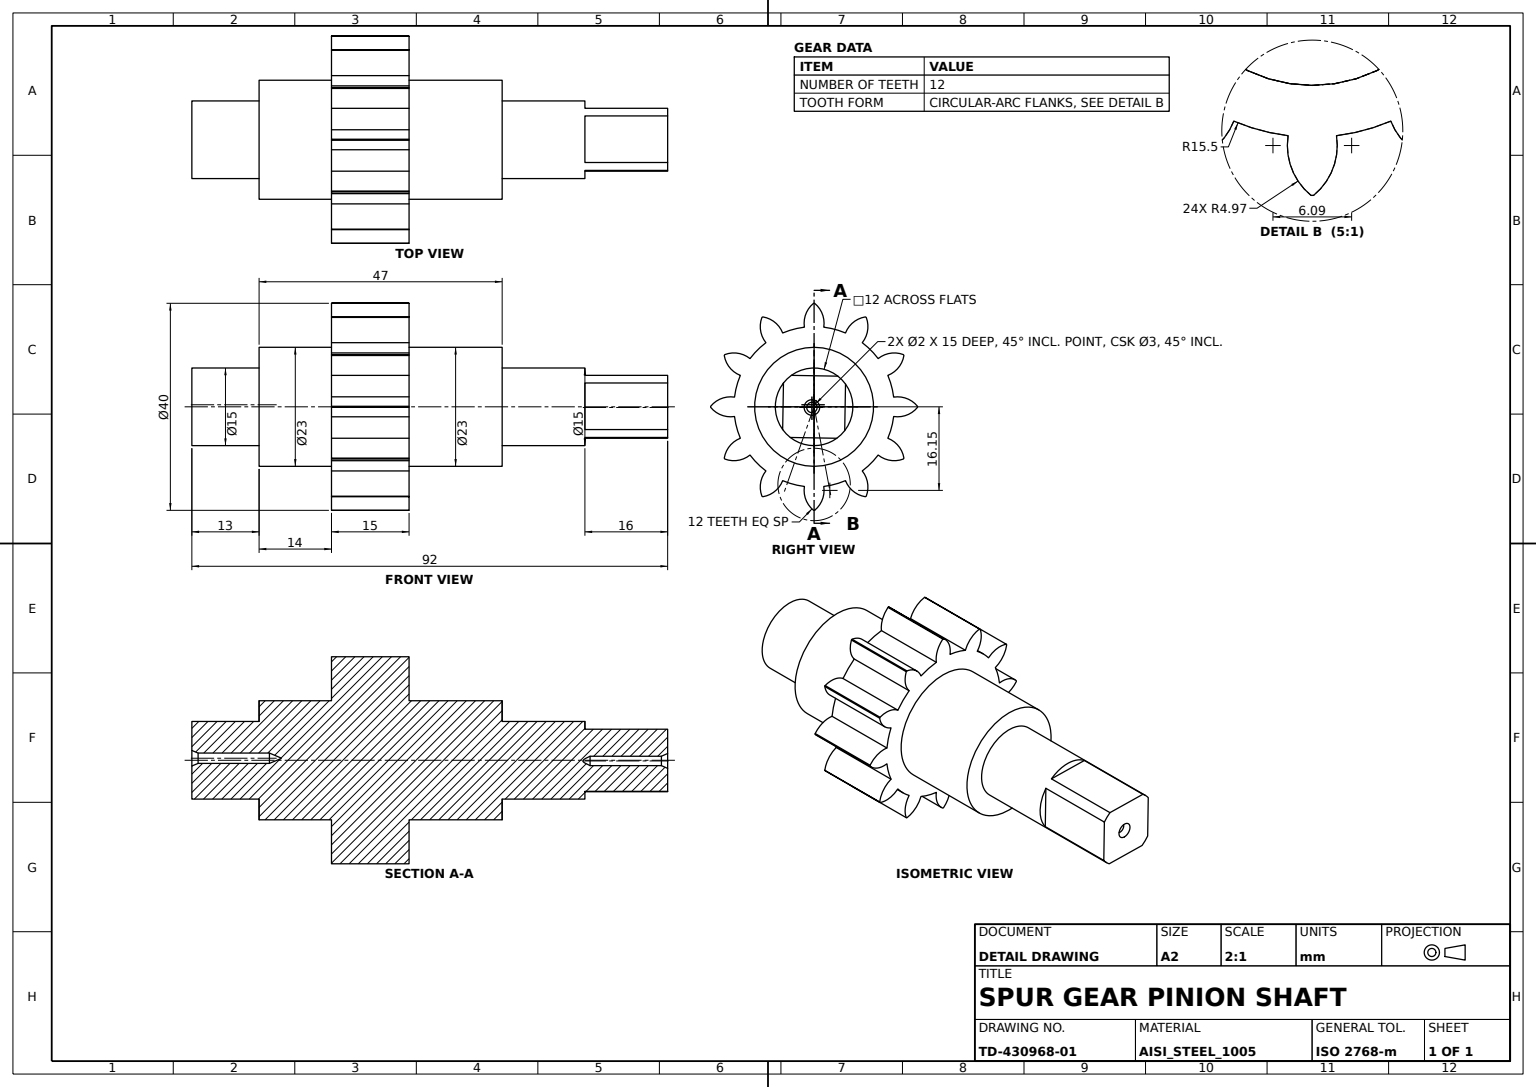
solid
v1 (0,-21.5,-11.5)
e1 v1 v1 CIRCLE(AX(P(0,-21.5,0),D(0,-1,0),D(0,0,-1)),11.5)
v2 (0,-7.5,-11.5)
e2 v2 v2 CIRCLE(AX(P(0,-7.5,0),D(0,-1,0),D(0,0,-1)),11.5)
face CYL(AX(P(0,0,0),D(0,-1,0),D(0,0,-1)),11.5) [-e1] [e2]
v3 (-1.87227,7.5,-15.386507)
v4 (-0.10064,7.5,-19.999747)
e3 v3 v4 CIRCLE(AX(P(3.042634,7.5,-16.14583),D(0,-1,0),D(1,0,0)),4.973213)
v5 (-0.10064,-7.5,-19.999747)
e4 v5 v4 LINE
v6 (-1.87227,-7.5,-15.386507)
e5 v6 v5 CIRCLE(AX(P(3.042634,-7.5,-16.14583),D(0,1,0),D(0,0,1)),4.973213) rev
e6 v3 v6 LINE
face CYL(AX(P(3.042634,-42.5,-16.14583),D(0,1,0),D(0,0,1)),4.973213) [e3 -e4 -e5 -e6]
v7 (14.261241,7.5,-6.071821)
v8 (15.386507,7.5,-1.87227)
e7 v7 v8 CIRCLE(AX(P(0,7.5,0),D(0,-1,0),D(1,0,0)),15.5)
v9 (15.386507,-7.5,-1.87227)
e8 v8 v9 LINE
v10 (14.261241,-7.5,-6.071821)
e9 v10 v9 CIRCLE(AX(P(0,-7.5,0),D(0,1,0),D(0,0,1)),15.5) rev
e10 v7 v10 LINE
face CYL(AX(P(0,-42.5,0),D(0,1,0),D(0,0,1)),15.5) [e7 e8 -e9 -e10]
v11 (0,-34.5,-7.5)
e11 v11 v11 CIRCLE(AX(P(0,-34.5,0),D(0,-1,0),D(0,0,-1)),7.5)
v12 (0,-21.5,-7.5)
e12 v12 v12 CIRCLE(AX(P(0,-21.5,0),D(0,-1,0),D(0,0,-1)),7.5)
face CYL(AX(P(0,0,0),D(0,-1,0),D(0,0,-1)),7.5) [-e11] [e12]
v13 (12.388971,7.5,9.314687)
v14 (9.314687,7.5,12.388971)
e13 v13 v14 CIRCLE(AX(P(0,7.5,0),D(0,-1,0),D(1,0,0)),15.5)
v15 (9.314687,-7.5,12.388971)
e14 v14 v15 LINE
v16 (12.388971,-7.5,9.314687)
e15 v16 v15 CIRCLE(AX(P(0,-7.5,0),D(0,1,0),D(0,0,1)),15.5) rev
e16 v13 v16 LINE
face CYL(AX(P(0,-42.5,0),D(0,1,0),D(0,0,1)),15.5) [e13 e14 -e15 -e16]
v17 (5.92055,41.5,4.604029)
v18 (5.92055,57.5,4.604029)
e17 v17 v18 LINE
v19 (6.077622,41.5,-4.3946)
e18 v17 v19 LINE
v20 (6.077622,57.5,-4.3946)
e19 v20 v19 LINE
e20 v20 v18 LINE
face PLANE(AX(P(6.077622,41.5,-4.3946),D(-0.999847695,0,-0.017452406),D(-0.017452406,0,0.999847695))) rev [-e17 e18 -e19 e20]
v21 (-9.912717,-7.5,17.370609)
v22 (-9.912717,7.5,17.370609)
e21 v21 v22 LINE
v23 (-6.071821,-7.5,14.261241)
e22 v23 v21 CIRCLE(AX(P(-10.707913,-7.5,12.461382),D(0,1,0),D(0,0,1)),4.973213) rev
v24 (-6.071821,7.5,14.261241)
e23 v24 v23 LINE
e24 v24 v22 CIRCLE(AX(P(-10.707913,7.5,12.461382),D(0,-1,0),D(-0.866025404,0,-0.5)),4.973213)
face CYL(AX(P(-10.707913,-42.5,12.461382),D(0,1,0),D(0,0,1)),4.973213) [-e21 -e22 -e23 e24]
v25 (-6.071821,7.5,-14.261241)
e25 v25 v3 CIRCLE(AX(P(0,7.5,0),D(0,-1,0),D(1,0,0)),15.5)
v26 (-6.071821,-7.5,-14.261241)
e26 v26 v6 CIRCLE(AX(P(0,-7.5,0),D(0,1,0),D(0,0,1)),15.5) rev
e27 v25 v26 LINE
face CYL(AX(P(0,-42.5,0),D(0,1,0),D(0,0,1)),15.5) [e25 e6 -e26 -e27]
v27 (9.314687,7.5,-12.388971)
v28 (9.314687,-7.5,-12.388971)
e28 v27 v28 LINE
v29 (10.08703,-7.5,-17.269969)
e29 v29 v28 CIRCLE(AX(P(5.437917,-7.5,-15.504016),D(0,1,0),D(0,0,1)),4.973213) rev
v30 (10.08703,7.5,-17.269969)
e30 v29 v30 LINE
e31 v30 v27 CIRCLE(AX(P(5.437917,7.5,-15.504016),D(0,-1,0),D(-0.866025404,0,-0.5)),4.973213)
face CYL(AX(P(5.437917,-42.5,-15.504016),D(0,1,0),D(0,0,1)),4.973213) [e28 -e29 e30 e31]
v31 (9.912717,7.5,17.370609)
v32 (6.071821,7.5,14.261241)
e32 v31 v32 CIRCLE(AX(P(10.707913,7.5,12.461382),D(0,-1,0),D(0.866025404,0,-0.5)),4.973213)
v33 (6.071821,-7.5,14.261241)
e33 v32 v33 LINE
v34 (9.912717,-7.5,17.370609)
e34 v34 v33 CIRCLE(AX(P(10.707913,-7.5,12.461382),D(0,1,0),D(0,0,1)),4.973213) rev
e35 v34 v31 LINE
face CYL(AX(P(10.707913,-42.5,12.461382),D(0,1,0),D(0,0,1)),4.973213) [e32 e33 -e34 e35]
v35 (0.421315,56.292893,-1.128229)
e36 v35 v35 CIRCLE(AX(P(0.421315,56.292893,-0.128229),D(0,-1,0),D(0,0,-1)),1) rev
v36 (0.421315,57.5,-1.628229)
e37 v36 v36 CIRCLE(AX(P(0.421315,57.5,-0.128229),D(0,-1,0),D(0,0,-1)),1.5)
face CONE(AX(P(0.421315,57.5,-0.128229),D(0,1,0),D(0,0,1)),1.5,0.392699082) rev [-e36] [-e37]
v37 (-14.261241,7.5,6.071821)
v38 (-14.261241,-7.5,6.071821)
e38 v37 v38 LINE
v39 (-17.370609,-7.5,9.912717)
e39 v39 v38 CIRCLE(AX(P(-12.461382,-7.5,10.707913),D(0,1,0),D(0,0,1)),4.973213) rev
v40 (-17.370609,7.5,9.912717)
e40 v39 v40 LINE
e41 v40 v37 CIRCLE(AX(P(-12.461382,7.5,10.707913),D(0,-1,0),D(0.5,0,0.866025404)),4.973213)
face CYL(AX(P(-12.461382,-42.5,10.707913),D(0,1,0),D(0,0,1)),4.973213) [e38 -e39 e40 e41]
v41 (1.87227,-7.5,15.386507)
v42 (0.10064,-7.5,19.999747)
e42 v41 v42 CIRCLE(AX(P(-3.042634,-7.5,16.14583),D(0,1,0),D(0,0,1)),4.973213) rev
v43 (1.87227,7.5,15.386507)
e43 v43 v41 LINE
v44 (0.10064,7.5,19.999747)
e44 v43 v44 CIRCLE(AX(P(-3.042634,7.5,16.14583),D(0,-1,0),D(-1,0,0)),4.973213)
e45 v42 v44 LINE
face CYL(AX(P(-3.042634,-42.5,16.14583),D(0,1,0),D(0,0,1)),4.973213) [-e42 -e43 e44 -e45]
v45 (0.043925,-19.5,1.395321)
e46 v45 v45 CIRCLE(AX(P(0.043925,-19.5,0.395321),D(0,1,0),D(0,0,1)),1) rev
v46 (0.043925,-33.292893,1.395321)
e47 v46 v46 CIRCLE(AX(P(0.043925,-33.292893,0.395321),D(0,1,0),D(0,0,1)),1) rev
face CYL(AX(P(0.043925,-19.5,0.395321),D(0,1,0),D(0,0,1)),1) rev [-e46] [e47]
v47 (19.999747,7.5,-0.10064)
e48 v8 v47 CIRCLE(AX(P(16.14583,7.5,3.042634),D(0,-1,0),D(0,0,1)),4.973213)
v48 (19.999747,-7.5,-0.10064)
e49 v48 v47 LINE
e50 v9 v48 CIRCLE(AX(P(16.14583,-7.5,3.042634),D(0,1,0),D(0,0,1)),4.973213) rev
face CYL(AX(P(16.14583,-42.5,3.042634),D(0,1,0),D(0,0,1)),4.973213) [-e8 e48 -e49 -e50]
v49 (-5.92055,41.5,-4.604029)
v50 (-6.077622,41.5,4.3946)
e51 v49 v50 LINE
e52 v49 v50 CIRCLE(AX(P(0,41.5,0),D(0,1,0),D(0,0,-1)),7.5)
face PLANE(AX(P(0,41.5,0),D(0,1,0),D(0,0,1))) [-e51 e52]
v51 (10.08703,-7.5,17.269969)
e53 v51 v34 CIRCLE(AX(P(0,-7.5,0),D(0,-1,0),D(0,0,-1)),20)
v52 (10.08703,7.5,17.269969)
e54 v51 v52 LINE
e55 v52 v31 CIRCLE(AX(P(0,7.5,0),D(0,-1,0),D(0,0,-1)),20)
face CYL(AX(P(0,0,0),D(0,-1,0),D(0,0,-1)),20) [-e35 -e53 e54 e55]
v53 (-4.604029,41.5,5.92055)
v54 (4.3946,41.5,6.077622)
e56 v53 v54 CIRCLE(AX(P(0,41.5,0),D(0,1,0),D(0,0,-1)),7.5)
e57 v53 v54 LINE
face PLANE(AX(P(0,41.5,0),D(0,1,0),D(0,0,1))) [e56 -e57]
v55 (-17.370609,-7.5,-9.912717)
v56 (-17.370609,7.5,-9.912717)
e58 v55 v56 LINE
v57 (-14.261241,-7.5,-6.071821)
e59 v57 v55 CIRCLE(AX(P(-12.461382,-7.5,-10.707913),D(0,1,0),D(0,0,1)),4.973213) rev
v58 (-14.261241,7.5,-6.071821)
e60 v58 v57 LINE
e61 v58 v56 CIRCLE(AX(P(-12.461382,7.5,-10.707913),D(0,-1,0),D(0.5,0,-0.866025404)),4.973213)
face CYL(AX(P(-12.461382,-42.5,-10.707913),D(0,1,0),D(0,0,1)),4.973213) [-e58 -e59 -e60 e61]
v59 (-10.08703,7.5,17.269969)
e62 v22 v59 CIRCLE(AX(P(0,7.5,0),D(0,-1,0),D(0,0,-1)),20)
v60 (-10.08703,-7.5,17.269969)
e63 v60 v59 LINE
e64 v21 v60 CIRCLE(AX(P(0,-7.5,0),D(0,-1,0),D(0,0,-1)),20)
face CYL(AX(P(0,0,0),D(0,-1,0),D(0,0,-1)),20) [e62 -e63 -e64 e21]
v61 (19.999747,-7.5,0.10064)
v62 (15.386507,-7.5,1.87227)
e65 v61 v62 CIRCLE(AX(P(16.14583,-7.5,-3.042634),D(0,1,0),D(0,0,1)),4.973213) rev
v63 (19.999747,7.5,0.10064)
e66 v61 v63 LINE
v64 (15.386507,7.5,1.87227)
e67 v63 v64 CIRCLE(AX(P(16.14583,7.5,-3.042634),D(0,-1,0),D(0,0,-1)),4.973213)
e68 v64 v62 LINE
face CYL(AX(P(16.14583,-42.5,-3.042634),D(0,1,0),D(0,0,1)),4.973213) [-e65 e66 e67 e68]
v65 (12.388971,-7.5,-9.314687)
e69 v28 v65 CIRCLE(AX(P(0,-7.5,0),D(0,1,0),D(0,0,1)),15.5) rev
v66 (17.269969,-7.5,-10.08703)
e70 v65 v66 CIRCLE(AX(P(15.504016,-7.5,-5.437917),D(0,1,0),D(0,0,1)),4.973213) rev
v67 (17.370609,-7.5,-9.912717)
e71 v66 v67 CIRCLE(AX(P(0,-7.5,0),D(0,-1,0),D(0,0,-1)),20)
e72 v67 v10 CIRCLE(AX(P(12.461382,-7.5,-10.707913),D(0,1,0),D(0,0,1)),4.973213) rev
e73 v48 v61 CIRCLE(AX(P(0,-7.5,0),D(0,-1,0),D(0,0,-1)),20)
v68 (14.261241,-7.5,6.071821)
e74 v62 v68 CIRCLE(AX(P(0,-7.5,0),D(0,1,0),D(0,0,1)),15.5) rev
v69 (17.370609,-7.5,9.912717)
e75 v68 v69 CIRCLE(AX(P(12.461382,-7.5,10.707913),D(0,1,0),D(0,0,1)),4.973213) rev
v70 (17.269969,-7.5,10.08703)
e76 v69 v70 CIRCLE(AX(P(0,-7.5,0),D(0,-1,0),D(0,0,-1)),20)
e77 v70 v16 CIRCLE(AX(P(15.504016,-7.5,5.437917),D(0,1,0),D(0,0,1)),4.973213) rev
e78 v15 v51 CIRCLE(AX(P(5.437917,-7.5,15.504016),D(0,1,0),D(0,0,1)),4.973213) rev
e79 v33 v41 CIRCLE(AX(P(0,-7.5,0),D(0,1,0),D(0,0,1)),15.5) rev
v71 (-0.10064,-7.5,19.999747)
e80 v42 v71 CIRCLE(AX(P(0,-7.5,0),D(0,-1,0),D(0,0,-1)),20)
v72 (-1.87227,-7.5,15.386507)
e81 v71 v72 CIRCLE(AX(P(3.042634,-7.5,16.14583),D(0,1,0),D(0,0,1)),4.973213) rev
e82 v72 v23 CIRCLE(AX(P(0,-7.5,0),D(0,1,0),D(0,0,1)),15.5) rev
v73 (-9.314687,-7.5,12.388971)
e83 v60 v73 CIRCLE(AX(P(-5.437917,-7.5,15.504016),D(0,1,0),D(0,0,1)),4.973213) rev
v74 (-12.388971,-7.5,9.314687)
e84 v73 v74 CIRCLE(AX(P(0,-7.5,0),D(0,1,0),D(0,0,1)),15.5) rev
v75 (-17.269969,-7.5,10.08703)
e85 v74 v75 CIRCLE(AX(P(-15.504016,-7.5,5.437917),D(0,1,0),D(0,0,1)),4.973213) rev
e86 v75 v39 CIRCLE(AX(P(0,-7.5,0),D(0,-1,0),D(0,0,-1)),20)
v76 (-15.386507,-7.5,1.87227)
e87 v38 v76 CIRCLE(AX(P(0,-7.5,0),D(0,1,0),D(0,0,1)),15.5) rev
v77 (-19.999747,-7.5,0.10064)
e88 v76 v77 CIRCLE(AX(P(-16.14583,-7.5,-3.042634),D(0,1,0),D(0,0,1)),4.973213) rev
v78 (-19.999747,-7.5,-0.10064)
e89 v77 v78 CIRCLE(AX(P(0,-7.5,0),D(0,-1,0),D(0,0,-1)),20)
v79 (-15.386507,-7.5,-1.87227)
e90 v78 v79 CIRCLE(AX(P(-16.14583,-7.5,3.042634),D(0,1,0),D(0,0,1)),4.973213) rev
e91 v79 v57 CIRCLE(AX(P(0,-7.5,0),D(0,1,0),D(0,0,1)),15.5) rev
v80 (-17.269969,-7.5,-10.08703)
e92 v55 v80 CIRCLE(AX(P(0,-7.5,0),D(0,-1,0),D(0,0,-1)),20)
v81 (-12.388971,-7.5,-9.314687)
e93 v80 v81 CIRCLE(AX(P(-15.504016,-7.5,-5.437917),D(0,1,0),D(0,0,1)),4.973213) rev
v82 (-9.314687,-7.5,-12.388971)
e94 v81 v82 CIRCLE(AX(P(0,-7.5,0),D(0,1,0),D(0,0,1)),15.5) rev
v83 (-10.08703,-7.5,-17.269969)
e95 v82 v83 CIRCLE(AX(P(-5.437917,-7.5,-15.504016),D(0,1,0),D(0,0,1)),4.973213) rev
v84 (-9.912717,-7.5,-17.370609)
e96 v83 v84 CIRCLE(AX(P(0,-7.5,0),D(0,-1,0),D(0,0,-1)),20)
e97 v84 v26 CIRCLE(AX(P(-10.707913,-7.5,-12.461382),D(0,1,0),D(0,0,1)),4.973213) rev
v85 (0.10064,-7.5,-19.999747)
e98 v5 v85 CIRCLE(AX(P(0,-7.5,0),D(0,-1,0),D(0,0,-1)),20)
v86 (1.87227,-7.5,-15.386507)
e99 v85 v86 CIRCLE(AX(P(-3.042634,-7.5,-16.14583),D(0,1,0),D(0,0,1)),4.973213) rev
v87 (6.071821,-7.5,-14.261241)
e100 v86 v87 CIRCLE(AX(P(0,-7.5,0),D(0,1,0),D(0,0,1)),15.5) rev
v88 (9.912717,-7.5,-17.370609)
e101 v87 v88 CIRCLE(AX(P(10.707913,-7.5,-12.461382),D(0,1,0),D(0,0,1)),4.973213) rev
e102 v88 v29 CIRCLE(AX(P(0,-7.5,0),D(0,-1,0),D(0,0,-1)),20)
face PLANE(AX(P(-20,-7.5,0),D(0,1,0),D(0,0,1))) rev [e69 e70 e71 e72 e9 e50 e73 e65 e74 e75 e76 e77 e15 e78 e53 e34 e79 e42 e80 e81 e82 e22 e64 e83 e84 e85 e86 e39 e87 e88 e89 e90 e91 e59 e92 e93 e94 e95 e96 e97 e26 e5 e98 e99 e100 e101 e102 e29] [-e2]
v89 (-6.077622,57.5,4.3946)
e103 v50 v89 LINE
v90 (-5.92055,57.5,-4.604029)
e104 v89 v90 LINE
e105 v90 v49 LINE
face PLANE(AX(P(-6.077622,41.5,4.3946),D(0.999847695,0,0.017452406),D(0.017452406,0,-0.999847695))) rev [e51 e103 e104 e105]
v91 (4.3946,57.5,6.077622)
e106 v54 v91 LINE
v92 (-4.604029,57.5,5.92055)
e107 v91 v92 LINE
e108 v92 v53 LINE
face PLANE(AX(P(4.3946,41.5,6.077622),D(0.017452406,0,-0.999847695),D(-0.999847695,0,-0.017452406))) rev [e57 e106 e107 e108]
v93 (17.269969,7.5,-10.08703)
e109 v66 v93 LINE
v94 (17.370609,7.5,-9.912717)
e110 v93 v94 CIRCLE(AX(P(0,7.5,0),D(0,-1,0),D(0,0,-1)),20)
e111 v67 v94 LINE
face CYL(AX(P(0,0,0),D(0,-1,0),D(0,0,-1)),20) [e109 e110 -e111 -e71]
v95 (17.269969,7.5,10.08703)
e112 v70 v95 LINE
e113 v95 v13 CIRCLE(AX(P(15.504016,7.5,5.437917),D(0,-1,0),D(0.5,0,-0.866025404)),4.973213)
face CYL(AX(P(15.504016,-42.5,5.437917),D(0,1,0),D(0,0,1)),4.973213) [e112 e113 e16 -e77]
v96 (0,25.5,-11.5)
e114 v96 v96 CIRCLE(AX(P(0,25.5,0),D(0,-1,0),D(0,0,-1)),11.5)
v97 (0,25.5,-7.5)
e115 v97 v97 CIRCLE(AX(P(0,25.5,0),D(0,-1,0),D(0,0,-1)),7.5)
face PLANE(AX(P(-7.5,25.5,0),D(0,-1,0),D(0,0,-1))) rev [-e114] [e115]
e116 v18 v91 CIRCLE(AX(P(0,57.5,0),D(0,-1,0),D(0,0,-1)),7.5)
v98 (4.604029,57.5,-5.92055)
e117 v98 v20 CIRCLE(AX(P(0,57.5,0),D(0,-1,0),D(0,0,-1)),7.5)
v99 (-4.3946,57.5,-6.077622)
e118 v99 v98 LINE
e119 v90 v99 CIRCLE(AX(P(0,57.5,0),D(0,-1,0),D(0,0,-1)),7.5)
e120 v92 v89 CIRCLE(AX(P(0,57.5,0),D(0,-1,0),D(0,0,-1)),7.5)
face PLANE(AX(P(0,57.5,0),D(0,-1,0),D(0,0,-1))) rev [-e107 -e116 -e20 -e117 -e118 -e119 -e104 -e120] [e37]
e121 v47 v63 CIRCLE(AX(P(0,7.5,0),D(0,-1,0),D(0,0,-1)),20)
face CYL(AX(P(0,0,0),D(0,-1,0),D(0,0,-1)),20) [e121 -e66 -e73 e49]
e122 v32 v43 CIRCLE(AX(P(0,7.5,0),D(0,-1,0),D(1,0,0)),15.5)
face CYL(AX(P(0,-42.5,0),D(0,1,0),D(0,0,1)),15.5) [e43 -e79 -e33 e122]
v100 (9.912717,7.5,-17.370609)
e123 v100 v30 CIRCLE(AX(P(0,7.5,0),D(0,-1,0),D(0,0,-1)),20)
e124 v88 v100 LINE
face CYL(AX(P(0,0,0),D(0,-1,0),D(0,0,-1)),20) [e123 -e30 -e102 e124]
v101 (-15.386507,7.5,1.87227)
e125 v101 v76 LINE
v102 (-19.999747,7.5,0.10064)
e126 v101 v102 CIRCLE(AX(P(-16.14583,7.5,-3.042634),D(0,-1,0),D(0,0,-1)),4.973213)
e127 v77 v102 LINE
face CYL(AX(P(-16.14583,-42.5,-3.042634),D(0,1,0),D(0,0,1)),4.973213) [-e88 -e125 e126 -e127]
v103 (1.87227,7.5,-15.386507)
e128 v103 v86 LINE
v104 (0.10064,7.5,-19.999747)
e129 v85 v104 LINE
e130 v104 v103 CIRCLE(AX(P(-3.042634,7.5,-16.14583),D(0,-1,0),D(-1,0,0)),4.973213)
face CYL(AX(P(-3.042634,-42.5,-16.14583),D(0,1,0),D(0,0,1)),4.973213) [e128 -e99 e129 e130]
v105 (-17.269969,7.5,10.08703)
e131 v75 v105 LINE
e132 v105 v40 CIRCLE(AX(P(0,7.5,0),D(0,-1,0),D(0,0,-1)),20)
face CYL(AX(P(0,0,0),D(0,-1,0),D(0,0,-1)),20) [-e86 e131 e132 -e40]
face PLANE(AX(P(-11.5,-21.5,0),D(0,1,0),D(0,0,1))) rev [e1] [-e12]
v106 (0.421315,42.5,-1.128229)
e133 v106 v106 CIRCLE(AX(P(0.421315,42.5,-0.128229),D(0,-1,0),D(0,0,-1)),1) rev
face CYL(AX(P(0.421315,42.5,-0.128229),D(0,-1,0),D(0,0,-1)),1) rev [-e133] [e36]
v107 (-4.3946,41.5,-6.077622)
e134 v99 v107 LINE
v108 (4.604029,41.5,-5.92055)
e135 v108 v107 CIRCLE(AX(P(0,41.5,0),D(0,1,0),D(0,0,-1)),7.5)
e136 v108 v98 LINE
e137 v17 v19 CIRCLE(AX(P(0,41.5,0),D(0,1,0),D(0,0,-1)),7.5)
face CYL(AX(P(0,0,0),D(0,-1,0),D(0,0,-1)),7.5) [e116 -e106 -e56 -e108 e120 -e103 -e52 -e105 e119 e134 -e135 e136 e117 e19 -e137 e17] [-e115]
v109 (-0.10064,7.5,19.999747)
v110 (-1.87227,7.5,15.386507)
e138 v109 v110 CIRCLE(AX(P(3.042634,7.5,16.14583),D(0,-1,0),D(1,0,0)),4.973213)
e139 v110 v72 LINE
e140 v71 v109 LINE
face CYL(AX(P(3.042634,-42.5,16.14583),D(0,1,0),D(0,0,1)),4.973213) [e138 e139 -e81 e140]
v111 (14.261241,7.5,6.071821)
v112 (17.370609,7.5,9.912717)
e141 v111 v112 CIRCLE(AX(P(12.461382,7.5,10.707913),D(0,-1,0),D(-0.5,0,0.866025404)),4.973213)
e142 v69 v112 LINE
e143 v111 v68 LINE
face CYL(AX(P(12.461382,-42.5,10.707913),D(0,1,0),D(0,0,1)),4.973213) [e141 -e142 -e75 -e143]
v113 (0.043925,-34.5,1.895321)
e144 v113 v113 CIRCLE(AX(P(0.043925,-34.5,0.395321),D(0,1,0),D(0,0,1)),1.5)
face CONE(AX(P(0.043925,-34.5,0.395321),D(0,-1,0),D(0,0,-1)),1.5,0.392699082) rev [-e47] [-e144]
v114 (0.043925,-17.085786,0.395321)
face CONE(AX(P(0.043925,-19.5,0.395321),D(0,-1,0),D(0,0,-1)),1,0.392699082) rev [e46] [v114]
v115 (-19.999747,7.5,-0.10064)
e145 v78 v115 LINE
v116 (-15.386507,7.5,-1.87227)
e146 v115 v116 CIRCLE(AX(P(-16.14583,7.5,3.042634),D(0,-1,0),D(0,0,1)),4.973213)
e147 v116 v79 LINE
face CYL(AX(P(-16.14583,-42.5,3.042634),D(0,1,0),D(0,0,1)),4.973213) [e145 e146 e147 -e90]
e148 v37 v101 CIRCLE(AX(P(0,7.5,0),D(0,-1,0),D(1,0,0)),15.5)
face CYL(AX(P(0,-42.5,0),D(0,1,0),D(0,0,1)),15.5) [-e38 e148 e125 -e87]
v117 (6.071821,7.5,-14.261241)
e149 v117 v87 LINE
e150 v117 v100 CIRCLE(AX(P(10.707913,7.5,-12.461382),D(0,-1,0),D(0.866025404,0,0.5)),4.973213)
face CYL(AX(P(10.707913,-42.5,-12.461382),D(0,1,0),D(0,0,1)),4.973213) [-e124 -e101 -e149 e150]
e151 v4 v104 CIRCLE(AX(P(0,7.5,0),D(0,-1,0),D(0,0,-1)),20)
face CYL(AX(P(0,0,0),D(0,-1,0),D(0,0,-1)),20) [e4 e151 -e129 -e98]
e152 v112 v95 CIRCLE(AX(P(0,7.5,0),D(0,-1,0),D(0,0,-1)),20)
face CYL(AX(P(0,0,0),D(0,-1,0),D(0,0,-1)),20) [-e76 e142 e152 -e112]
v118 (0,7.5,-11.5)
e153 v118 v118 CIRCLE(AX(P(0,7.5,0),D(0,-1,0),D(0,0,-1)),11.5)
face CYL(AX(P(0,0,0),D(0,-1,0),D(0,0,-1)),11.5) [e114] [-e153]
e154 v102 v115 CIRCLE(AX(P(0,7.5,0),D(0,-1,0),D(0,0,-1)),20)
face CYL(AX(P(0,0,0),D(0,-1,0),D(0,0,-1)),20) [-e145 -e89 e127 e154]
v119 (-10.08703,7.5,-17.269969)
e155 v83 v119 LINE
v120 (-9.912717,7.5,-17.370609)
e156 v119 v120 CIRCLE(AX(P(0,7.5,0),D(0,-1,0),D(0,0,-1)),20)
e157 v84 v120 LINE
face CYL(AX(P(0,0,0),D(0,-1,0),D(0,0,-1)),20) [e155 e156 -e157 -e96]
v121 (12.388971,7.5,-9.314687)
e158 v121 v65 LINE
e159 v27 v121 CIRCLE(AX(P(0,7.5,0),D(0,-1,0),D(1,0,0)),15.5)
face CYL(AX(P(0,-42.5,0),D(0,1,0),D(0,0,1)),15.5) [e158 -e69 -e28 e159]
e160 v110 v24 CIRCLE(AX(P(0,7.5,0),D(0,-1,0),D(1,0,0)),15.5)
face CYL(AX(P(0,-42.5,0),D(0,1,0),D(0,0,1)),15.5) [e160 e23 -e82 -e139]
v122 (-12.388971,7.5,9.314687)
e161 v122 v105 CIRCLE(AX(P(-15.504016,7.5,5.437917),D(0,-1,0),D(-0.5,0,-0.866025404)),4.973213)
v123 (-9.314687,7.5,12.388971)
e162 v123 v122 CIRCLE(AX(P(0,7.5,0),D(0,-1,0),D(1,0,0)),15.5)
e163 v59 v123 CIRCLE(AX(P(-5.437917,7.5,15.504016),D(0,-1,0),D(0.866025404,0,0.5)),4.973213)
e164 v44 v109 CIRCLE(AX(P(0,7.5,0),D(0,-1,0),D(0,0,-1)),20)
e165 v14 v52 CIRCLE(AX(P(5.437917,7.5,15.504016),D(0,-1,0),D(-0.866025404,0,0.5)),4.973213)
e166 v64 v111 CIRCLE(AX(P(0,7.5,0),D(0,-1,0),D(1,0,0)),15.5)
e167 v94 v7 CIRCLE(AX(P(12.461382,7.5,-10.707913),D(0,-1,0),D(-0.5,0,-0.866025404)),4.973213)
e168 v121 v93 CIRCLE(AX(P(15.504016,7.5,-5.437917),D(0,-1,0),D(0.5,0,0.866025404)),4.973213)
e169 v103 v117 CIRCLE(AX(P(0,7.5,0),D(0,-1,0),D(1,0,0)),15.5)
e170 v120 v25 CIRCLE(AX(P(-10.707913,7.5,-12.461382),D(0,-1,0),D(-0.866025404,0,0.5)),4.973213)
v124 (-9.314687,7.5,-12.388971)
e171 v124 v119 CIRCLE(AX(P(-5.437917,7.5,-15.504016),D(0,-1,0),D(0.866025404,0,-0.5)),4.973213)
v125 (-12.388971,7.5,-9.314687)
e172 v125 v124 CIRCLE(AX(P(0,7.5,0),D(0,-1,0),D(1,0,0)),15.5)
v126 (-17.269969,7.5,-10.08703)
e173 v126 v125 CIRCLE(AX(P(-15.504016,7.5,-5.437917),D(0,-1,0),D(-0.5,0,0.866025404)),4.973213)
e174 v56 v126 CIRCLE(AX(P(0,7.5,0),D(0,-1,0),D(0,0,-1)),20)
e175 v116 v58 CIRCLE(AX(P(0,7.5,0),D(0,-1,0),D(1,0,0)),15.5)
face PLANE(AX(P(-11.5,7.5,0),D(0,-1,0),D(0,0,-1))) rev [e153] [-e154 -e126 -e148 -e41 -e132 -e161 -e162 -e163 -e62 -e24 -e160 -e138 -e164 -e44 -e122 -e32 -e55 -e165 -e13 -e113 -e152 -e141 -e166 -e67 -e121 -e48 -e7 -e167 -e110 -e168 -e159 -e31 -e123 -e150 -e169 -e130 -e151 -e3 -e25 -e170 -e156 -e171 -e172 -e173 -e174 -e61 -e175 -e146]
face CYL(AX(P(0,-42.5,0),D(0,1,0),D(0,0,1)),15.5) [-e68 e166 e143 -e74]
face CYL(AX(P(0,-42.5,0),D(0,1,0),D(0,0,1)),15.5) [-e147 e175 e60 -e91]
v127 (0.421315,40.085786,-0.128229)
face CONE(AX(P(0.421315,42.5,-0.128229),D(0,1,0),D(0,0,1)),1,0.392699082) rev [v127] [e133]
e176 v122 v74 LINE
face CYL(AX(P(-15.504016,-42.5,5.437917),D(0,1,0),D(0,0,1)),4.973213) [-e131 -e85 -e176 e161]
e177 v108 v107 LINE
face PLANE(AX(P(0,41.5,0),D(0,1,0),D(0,0,1))) [-e177 e135]
face CYL(AX(P(12.461382,-42.5,-10.707913),D(0,1,0),D(0,0,1)),4.973213) [e167 e10 -e72 e111]
e178 v123 v73 LINE
face CYL(AX(P(-5.437917,-42.5,15.504016),D(0,1,0),D(0,0,1)),4.973213) [e63 e163 e178 -e83]
face CYL(AX(P(0,-42.5,0),D(0,1,0),D(0,0,1)),15.5) [-e178 e162 e176 -e84]
face PLANE(AX(P(0,41.5,0),D(0,1,0),D(0,0,1))) [-e18 e137]
e179 v80 v126 LINE
face CYL(AX(P(0,0,0),D(0,-1,0),D(0,0,-1)),20) [e174 -e179 -e92 e58]
face PLANE(AX(P(-7.5,-34.5,0),D(0,1,0),D(0,0,1))) rev [e144] [e11]
face CYL(AX(P(15.504016,-42.5,-5.437917),D(0,1,0),D(0,0,1)),4.973213) [-e158 e168 -e109 -e70]
e180 v125 v81 LINE
e181 v124 v82 LINE
face CYL(AX(P(0,-42.5,0),D(0,1,0),D(0,0,1)),15.5) [-e94 -e180 e172 e181]
face PLANE(AX(P(-4.3946,41.5,-6.077622),D(-0.017452406,0,0.999847695),D(0.999847695,0,0.017452406))) rev [-e134 e118 -e136 e177]
face CYL(AX(P(0,0,0),D(0,-1,0),D(0,0,-1)),20) [e164 -e140 -e80 e45]
face CYL(AX(P(0,-42.5,0),D(0,1,0),D(0,0,1)),15.5) [e149 -e100 -e128 e169]
face CYL(AX(P(-5.437917,-42.5,-15.504016),D(0,1,0),D(0,0,1)),4.973213) [-e155 -e95 -e181 e171]
face CYL(AX(P(-15.504016,-42.5,-5.437917),D(0,1,0),D(0,0,1)),4.973213) [e173 e180 -e93 e179]
face CYL(AX(P(5.437917,-42.5,15.504016),D(0,1,0),D(0,0,1)),4.973213) [e165 -e54 -e78 -e14]
face CYL(AX(P(-10.707913,-42.5,-12.461382),D(0,1,0),D(0,0,1)),4.973213) [e157 e170 e27 -e97]
